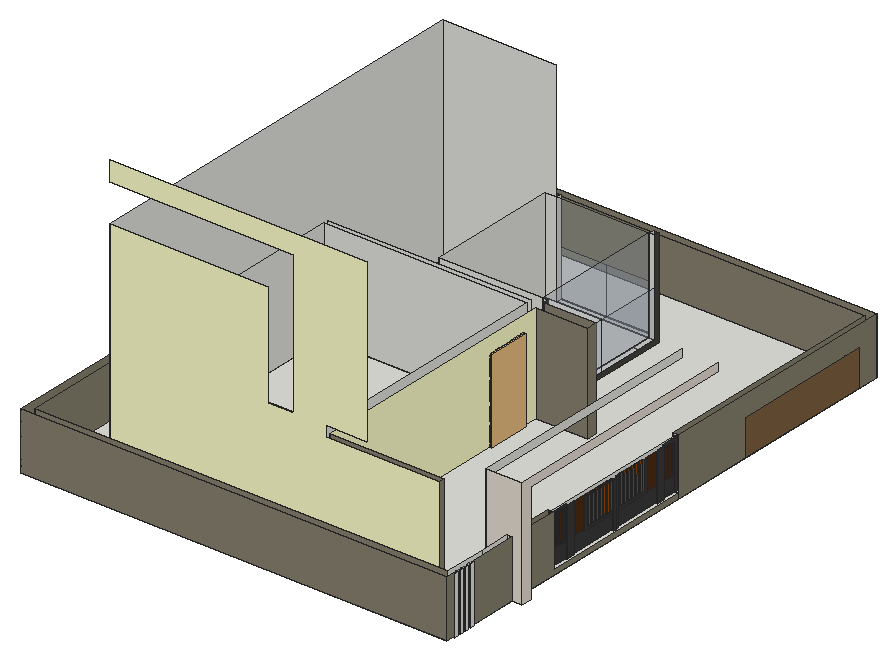
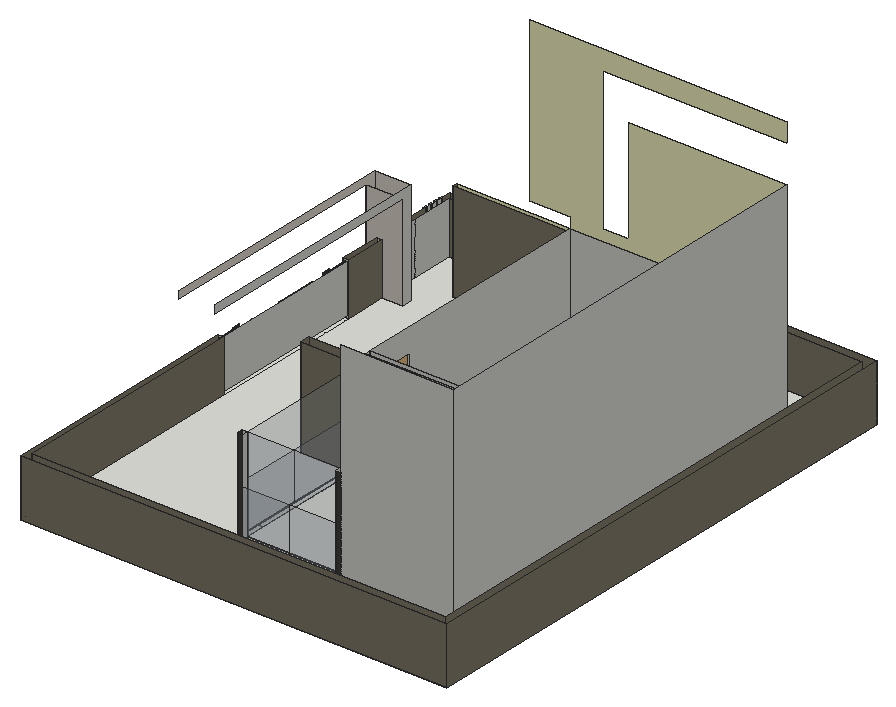
# SketchUp Ruby script. Lengths in inches.
U = 1.inch
M = Sketchup.active_model
def pt(a) = Geom::Point3d.new(a.map { |v| v * U })
def face(e, loops, mat)
  f = e.add_face(loops[0].map { |a| pt(a) })
  loops[1..].each { |l| e.add_face(l.map { |a| pt(a) }).erase! }
  f.material = f.back_material = mat if mat
  f
end
# faces: each face lists its corners as indices into pts; further lists are holes
def faces(e, pts, list, mat = nil) = list.each { |f| face(e, (f[0].is_a?(Array) ? f : [f]).map { |l| l.map { |i| pts[i] } }, mat) }
# xy, xz, yz: faces in a plane at the given z, y or x. An outline is a flat list of corners, or four numbers for a rectangle; further outlines are holes
def ring(l) = l.size == 4 ? [[l[0], l[1]], [l[2], l[1]], [l[2], l[3]], [l[0], l[3]]] : l.each_slice(2).to_a
def flat(e, list, mat, &to3) = list.each { |f| face(e, (f[0].is_a?(Array) ? f : [f]).map { |l| ring(l).map { |u, v| to3.(u, v) } }, mat) }
def xy(e, z, list, mat = nil) = flat(e, list, mat) { |x, y| [x, y, z] }
def xz(e, y, list, mat = nil) = flat(e, list, mat) { |x, z| [x, y, z] }
def yz(e, x, list, mat = nil) = flat(e, list, mat) { |y, z| [x, y, z] }
def lines(e, pts, list) = list.each { |a, b| e.add_line(pt(pts[a]), pt(pts[b])) }
# prism: a flat outline (further loops are holes) pulled along v
def prism(e, loops, v, mat = nil)
  f = face(e, loops, mat); d = Geom::Vector3d.new(v.map { |x| x * U })
  f.pushpull(f.normal.samedirection?(d) ? d.length : -d.length)
end
def box(e, o, s, mat = nil) = prism(e, [[o, [o[0] + s[0], o[1], o[2]], [o[0] + s[0], o[1] + s[1], o[2]], [o[0], o[1] + s[1], o[2]]]], [0, 0, s[2]], mat)
def at(x, y, z, deg = 0) = Geom::Transformation.translation(pt([x, y, z])) * Geom::Transformation.rotation(ORIGIN, Z_AXIS, deg.degrees)
def axes(o, x, y, z) = Geom::Transformation.new([*x, 0, *y, 0, *z, 0, *pt(o).to_a, 1])
def part(name) = M.definitions.add(name)
# library, detail: a bought-in or finely detailed component or shape, given as its bounding box
def library(name, o, s) = part(name).tap { |d| box(d.entities, o, s) }
def detail(e, o, s) = box(e.add_group.entities, o, s)
def put(e, d, t, mat = nil) = e.add_instance(d, t).tap { |i| i.material = mat if mat }
def group(e, t, mat = nil) = e.add_group.tap { |g| g.transformation = t; g.material = mat if mat }.entities
root = M.entities
M.materials.add("Brick_09_1K").color = [135, 129, 110]
M.materials.add("C07_Caramel_Shine").color = [153, 76, 0]
M.materials.add("E01_Mint_Frost").color = [255, 255, 204]
M.materials.add("Glass_Basic_01").color = [161, 173, 186]
M.materials["Glass_Basic_01"].alpha = 0.25
M.materials.add("Marble_01_1K").color = [230, 221, 211]
M.materials.add("Plywood_01_1K").color = [125, 96, 64]
M.materials.add("Wood_Planks_01_1K").color = [69, 67, 63]
M.materials.add("[Color_007]1").color = [58, 58, 58]
M.materials.add("[Wood_Cherry_Original]1").color = [76, 43, 21]
c1 = library("porta+4",[0.2,-5.42,1.33],[46.55,4.72,83.21])
xy(root,-6,[[0,0,0,618.14,492,618.14,492,35.25,494,35.25,494,31.5,492,31.5,492,27.75,494,27.75,494,24,492,24,492,20.25,494,20.25,494,16.5,492,16.5,492,12.75,494,12.75,494,9,492,9,492,0],[492,93,504,105]])
xy(root,0,[[[9,9,486,9,486,93,462,93,462,105,486,105,486,609.14,9,609.14],[57,57,57,537,306,537,306,372,366,372,366,360,306,360,306,63,438,63,438,57]],[[57,57,306,57,306,360,366,360,366,372,306,372,306,537,300,537,300,360,66,360,66,537,57,537],[66,66,300,354]],[66,66,300,354],[486,153,492,333],[66,360,300,537]])
xy(root,2,[[488,153,488,333,490,333,490,312.5,492,312.5,492,303.5,490,303.5,490,246,492,246,492,240,490,240,490,182.5,492,182.5,492,173.5,490,173.5,490,153]],"[Color_007]1")
xy(root,3,[[300,297,306,339]])
xy(root,6,[[180,378,300,531],[300,378,306,508.51],[300,508.51,306,531],[193.5,531,300,537]])
xy(root,9,[[210,360,252,378]])
xy(root,20,[[488,155,490,155.93],[488,156.85,490,157.78],[488,158.7,490,159.625],[488,160.55,490,161.48],[488,162.4,490,163.33],
  [488,164.25,490,165.18],[488,166.1,490,167.03],[488,167.95,490,168.875],[488,169.8,490,170.73],[488,171.65,490,172.58],
  [488,315.28,490,316.2],[488,317.125,490,318.05],[488,318.98,490,319.9],[488,320.83,490,321.75],[488,322.68,490,323.6],
  [488,324.53,490,325.45],[488,326.375,490,327.3],[488,328.23,490,329.15],[488,330.08,490,331]])
xy(root,20,[[490,198,492,240],[490,246,492,288]],"[Color_007]1")
xy(root,23,[[488,201.98,492,202.95],[488,203.92,492,204.9],[488,205.875,492,206.85],[488,207.83,492,208.8],[488,209.78,492,210.75],
  [488,211.73,492,212.7],[488,213.68,492,214.65],[488,215.625,492,216.6],[488,217.58,492,218.55],[488,219.53,492,220.5],
  [488,221.48,492,222.45],[488,223.42,492,224.4],[488,225.375,492,226.35],[488,227.33,492,228.3],[488,229.28,492,230.25],
  [488,231.23,492,232.2],[488,233.18,492,234.15],[488,235.125,492,236.1],[488,237.08,492,238.05],[488,239.03,492,240],
  [488,246,492,246.98],[488,247.95,492,248.92],[488,249.9,492,250.875],[488,251.85,492,252.83],[488,253.8,492,254.78],
  [488,255.75,492,256.73],[488,257.7,492,258.68],[488,259.65,492,260.625],[488,261.6,492,262.58],[488,263.55,492,264.53],
  [488,265.5,492,266.48],[488,267.45,492,268.42],[488,269.4,492,270.375],[488,271.35,492,272.33],[488,273.3,492,274.28],
  [488,275.25,492,276.23],[488,277.2,492,278.18],[488,279.15,492,280.125],[488,281.1,492,282.08],[488,283.05,492,284.03]])
xy(root,23,[[490,201,492,201.98],[490,202.95,492,203.92],[490,204.9,492,205.875],[490,206.85,492,207.83],[490,208.8,492,209.78],
  [490,210.75,492,211.73],[490,212.7,492,213.68],[490,214.65,492,215.625],[490,216.6,492,217.58],[490,218.55,492,219.53],
  [490,220.5,492,221.48],[490,222.45,492,223.42],[490,224.4,492,225.375],[490,226.35,492,227.33],[490,228.3,492,229.28],
  [490,230.25,492,231.23],[490,232.2,492,233.18],[490,234.15,492,235.125],[490,236.1,492,237.08],[490,238.05,492,239.03],
  [490,246.98,492,247.95],[490,248.92,492,249.9],[490,250.875,492,251.85],[490,252.83,492,253.8],[490,254.78,492,255.75],
  [490,256.73,492,257.7],[490,258.68,492,259.65],[490,260.625,492,261.6],[490,262.58,492,263.55],[490,264.53,492,265.5],
  [490,266.48,492,267.45],[490,268.42,492,269.4],[490,270.375,492,271.35],[490,272.33,492,273.3],[490,274.28,492,275.25],
  [490,276.23,492,277.2],[490,278.18,492,279.15],[490,280.125,492,281.1],[490,282.08,492,283.05],[490,284.03,492,285]],"[Color_007]1")
xz(root,0,[[0,-6,492,60]],"Brick_09_1K")
xz(root,9,[[492,-6,494,60]])
xz(root,9,[[9,0,486,60]],"Brick_09_1K")
xz(root,12.75,[[492,-6,494,60]])
xz(root,16.5,[[492,-6,494,60]])
xz(root,20.25,[[492,-6,494,60]])
xz(root,24,[[492,-6,494,60]])
xz(root,27.75,[[492,-6,494,60]])
xz(root,31.5,[[492,-6,494,60]])
xz(root,35.25,[[492,-6,494,60]])
xz(root,57,[[57,0,438,0,438,114,306,114,306,126,354,126,354,312,57,312,57,289.5,270,289.5,270,126,240,126,240,246,57,246]],"E01_Mint_Frost")
xz(root,63,[[306,0,438,114]],"Brick_09_1K")
xz(root,66,[[66,0,300,120]])
xz(root,93,[[492,-6,504,-6,504,120,462,120,462,0,486,0,486,60,492,60]],"Marble_01_1K")
xz(root,105,[[492,-6,492,60,486,60,486,0,462,0,462,111,504,111,504,-6]],"Marble_01_1K")
xz(root,153,[[[486,0,492,60],[488,2,490,58]]])
xz(root,155,[[488,20,490,22],[488,22,490,55.99]])
xz(root,155.93,[[488,20,490,22],[488,22,490,55.98]])
xz(root,156.85,[[488,20,490,22],[488,22,490,55.98]])
xz(root,157.78,[[488,20,490,22],[488,22,490,55.97]])
xz(root,158.7,[[488,20,490,22],[488,22,490,55.97]])
xz(root,159.625,[[488,20,490,22],[488,22,490,55.96]])
xz(root,160.55,[[488,20,490,22],[488,22,490,55.96]])
xz(root,161.48,[[488,20,490,22],[488,22,490,55.95]])
xz(root,162.4,[[488,20,490,22],[488,22,490,55.95]])
xz(root,163.33,[[488,20,490,22.01],[488,22.01,490,55.94]])
xz(root,164.25,[[488,20,490,22.01],[488,22.01,490,55.9375]])
xz(root,165.18,[[488,20,490,22.01],[488,22.01,490,55.93]])
xz(root,166.1,[[488,20,490,22.01],[488,22.01,490,55.93]])
xz(root,167.03,[[488,20,490,22.01],[488,22.01,490,55.92]])
xz(root,167.95,[[488,20,490,22.01],[488,22.01,490,55.92]])
xz(root,168.875,[[488,20,490,22.01],[488,22.01,490,55.91]])
xz(root,169.8,[[488,20,490,22.01],[488,22.01,490,55.91]])
xz(root,170.73,[[488,20,490,22.01],[488,22.01,490,55.9]])
xz(root,171.65,[[488,20,490,22.01],[488,22.01,490,55.9]])
xz(root,172.58,[[488,20,490,22.01],[488,22.01,490,55.89]])
xz(root,173.5,[[490,2,492,20],[490,20,492,22],[490,22,492,58]],"[Color_007]1")
xz(root,182.5,[[490,2,492,55.84]],"[Color_007]1")
xz(root,198,[[490,20,492,55.75]],"[Color_007]1")
xz(root,201,[[490,23,492,55]],"[Color_007]1")
xz(root,201.98,[[488,23,490,55]],"[Color_007]1")
xz(root,202.95,[[488,23,490,55]],"[Color_007]1")
xz(root,203.92,[[488,23,490,55]],"[Color_007]1")
xz(root,204.9,[[488,23,490,55]],"[Color_007]1")
xz(root,205.875,[[488,23,490,55]],"[Color_007]1")
xz(root,206.85,[[488,23,490,55]],"[Color_007]1")
xz(root,207.83,[[488,23,490,55]],"[Color_007]1")
xz(root,208.8,[[488,23,490,55]],"[Color_007]1")
xz(root,209.78,[[488,23,490,55]],"[Color_007]1")
xz(root,210.75,[[488,23,490,55]],"[Color_007]1")
xz(root,211.73,[[488,23,490,55]],"[Color_007]1")
xz(root,212.7,[[488,23,490,55]],"[Color_007]1")
xz(root,213.68,[[488,23,490,55]],"[Color_007]1")
xz(root,214.65,[[488,23,490,55]],"[Color_007]1")
xz(root,215.625,[[488,23,490,55]],"[Color_007]1")
xz(root,216.6,[[488,23,490,55]],"[Color_007]1")
xz(root,217.58,[[488,23,490,55]],"[Color_007]1")
xz(root,218.55,[[488,23,490,55]],"[Color_007]1")
xz(root,219.53,[[488,23,490,55]],"[Color_007]1")
xz(root,220.5,[[488,23,490,55]],"[Color_007]1")
xz(root,221.48,[[488,23,490,55]],"[Color_007]1")
xz(root,222.45,[[488,23,490,55]],"[Color_007]1")
xz(root,223.42,[[488,23,490,55]],"[Color_007]1")
xz(root,224.4,[[488,23,490,55]],"[Color_007]1")
xz(root,225.375,[[488,23,490,55]],"[Color_007]1")
xz(root,226.35,[[488,23,490,55]],"[Color_007]1")
xz(root,227.33,[[488,23,490,55]],"[Color_007]1")
xz(root,228.3,[[488,23,490,55]],"[Color_007]1")
xz(root,229.28,[[488,23,490,55]],"[Color_007]1")
xz(root,230.25,[[488,23,490,55]],"[Color_007]1")
xz(root,231.23,[[488,23,490,55]],"[Color_007]1")
xz(root,232.2,[[488,23,490,55]],"[Color_007]1")
xz(root,233.18,[[488,23,490,55]],"[Color_007]1")
xz(root,234.15,[[488,23,490,55]],"[Color_007]1")
xz(root,235.125,[[488,23,490,55]],"[Color_007]1")
xz(root,236.1,[[488,23,490,55]],"[Color_007]1")
xz(root,237.08,[[488,23,490,55]],"[Color_007]1")
xz(root,238.05,[[488,23,490,55]],"[Color_007]1")
xz(root,239.03,[[488,23,490,55]])
xz(root,240,[[490,2,492,20],[488,23,492,55]],"[Color_007]1")
xz(root,246,[[490,2,492,20],[488,23,492,55]],"[Color_007]1")
xz(root,246.98,[[488,23,490,55]])
xz(root,247.95,[[488,23,490,55]],"[Color_007]1")
xz(root,248.92,[[488,23,490,55]],"[Color_007]1")
xz(root,249.9,[[488,23,490,55]],"[Color_007]1")
xz(root,250.875,[[488,23,490,55]],"[Color_007]1")
xz(root,251.85,[[488,23,490,55]],"[Color_007]1")
xz(root,252.83,[[488,23,490,55]],"[Color_007]1")
xz(root,253.8,[[488,23,490,55]],"[Color_007]1")
xz(root,254.78,[[488,23,490,55]],"[Color_007]1")
xz(root,255.75,[[488,23,490,55]],"[Color_007]1")
xz(root,256.73,[[488,23,490,55]],"[Color_007]1")
xz(root,257.7,[[488,23,490,55]],"[Color_007]1")
xz(root,258.68,[[488,23,490,55]],"[Color_007]1")
xz(root,259.65,[[488,23,490,55]],"[Color_007]1")
xz(root,260.625,[[488,23,490,55]],"[Color_007]1")
xz(root,261.6,[[488,23,490,55]],"[Color_007]1")
xz(root,262.58,[[488,23,490,55]],"[Color_007]1")
xz(root,263.55,[[488,23,490,55]],"[Color_007]1")
xz(root,264.53,[[488,23,490,55]],"[Color_007]1")
xz(root,265.5,[[488,23,490,55]],"[Color_007]1")
xz(root,266.48,[[488,23,490,55]],"[Color_007]1")
xz(root,267.45,[[488,23,490,55]],"[Color_007]1")
xz(root,268.42,[[488,23,490,55]],"[Color_007]1")
xz(root,269.4,[[488,23,490,55]],"[Color_007]1")
xz(root,270.375,[[488,23,490,55]],"[Color_007]1")
xz(root,271.35,[[488,23,490,55]],"[Color_007]1")
xz(root,272.33,[[488,23,490,55]],"[Color_007]1")
xz(root,273.3,[[488,23,490,55]],"[Color_007]1")
xz(root,274.28,[[488,23,490,55]],"[Color_007]1")
xz(root,275.25,[[488,23,490,55]],"[Color_007]1")
xz(root,276.23,[[488,23,490,55]],"[Color_007]1")
xz(root,277.2,[[488,23,490,55]],"[Color_007]1")
xz(root,278.18,[[488,23,490,55]],"[Color_007]1")
xz(root,279.15,[[488,23,490,55]],"[Color_007]1")
xz(root,280.125,[[488,23,490,55]],"[Color_007]1")
xz(root,281.1,[[488,23,490,55]],"[Color_007]1")
xz(root,282.08,[[488,23,490,55]],"[Color_007]1")
xz(root,283.05,[[488,23,490,55]],"[Color_007]1")
xz(root,284.03,[[488,23,490,55]],"[Color_007]1")
xz(root,285,[[490,23,492,55]],"[Color_007]1")
xz(root,288,[[490,20,492,55]],"[Color_007]1")
xz(root,297,[[300,3,306,93]])
xz(root,303.5,[[490,2,492,4],[490,4,492,20],[490,20,492,55.16]],"[Color_007]1")
xz(root,312.5,[[490,2,492,58]],"[Color_007]1")
xz(root,313.42,[[488,20.01,490,20.1]])
xz(root,313.42,[[488,20.1,490,55]],"[Color_007]1")
xz(root,314.35,[[488,20,490,20.1]])
xz(root,314.35,[[488,20.1,490,55]],"[Color_007]1")
xz(root,315.28,[[488,20,490,20.1]])
xz(root,315.28,[[488,20.1,490,55]],"[Color_007]1")
xz(root,316.2,[[488,20,490,20.1]])
xz(root,316.2,[[488,20.1,490,54.98]],"[Color_007]1")
xz(root,317.125,[[488,20,490,20.1]])
xz(root,317.125,[[488,20.1,490,54.98]],"[Color_007]1")
xz(root,318.05,[[488,20,490,20.1]])
xz(root,318.05,[[488,20.1,490,54.98]],"[Color_007]1")
xz(root,318.98,[[488,20,490,20.1]])
xz(root,318.98,[[488,20.1,490,54.98]],"[Color_007]1")
xz(root,319.9,[[488,20,490,20.1]])
xz(root,319.9,[[488,20.1,490,54.98]],"[Color_007]1")
xz(root,320.83,[[488,20,490,20.1]])
xz(root,320.83,[[488,20.1,490,54.98]],"[Color_007]1")
xz(root,321.75,[[488,20,490,20.1]])
xz(root,321.75,[[488,20.1,490,54.98]],"[Color_007]1")
xz(root,322.68,[[488,20,490,20.1]])
xz(root,322.68,[[488,20.1,490,54.98]],"[Color_007]1")
xz(root,323.6,[[488,20,490,20.1]])
xz(root,323.6,[[488,20.1,490,54.98]],"[Color_007]1")
xz(root,324.53,[[488,20,490,20.1]])
xz(root,324.53,[[488,20.1,490,54.98]],"[Color_007]1")
xz(root,325.45,[[488,20,490,20.1]])
xz(root,325.45,[[488,20.1,490,54.98]],"[Color_007]1")
xz(root,326.375,[[488,20,490,20.1]])
xz(root,326.375,[[488,20.1,490,54.98]],"[Color_007]1")
xz(root,327.3,[[488,20,490,20.1]])
xz(root,327.3,[[488,20.1,490,54.98]],"[Color_007]1")
xz(root,328.23,[[488,20,490,20.1]])
xz(root,328.23,[[488,20.1,490,54.98]],"[Color_007]1")
xz(root,329.15,[[488,20,490,20.1]])
xz(root,329.15,[[488,20.1,490,54.98]],"[Color_007]1")
xz(root,330.08,[[488,20,490,20.1]])
xz(root,330.08,[[488,20.1,490,54.98]],"[Color_007]1")
xz(root,331,[[488,20,490,20.1]])
xz(root,331,[[488,20.1,490,54.98]],"[Color_007]1")
xz(root,333,[[[486,0,492,60],[488,2,490,58]]])
xz(root,339,[[300,3,306,93]])
xz(root,354,[[66,0,300,120]])
xz(root,360,[[[66,0,300,120],[210,9,252,87]]])
xz(root,360,[[306,0,366,114]],"Brick_09_1K")
xz(root,372,[[306,0,366,114]],"Brick_09_1K")
xz(root,378,[[180,6,180,114,300,114,300,6,255,6,255,90,207,90,207,6],[[207,6,255,90],[210,9,252,87]],[300,6,306,114]])
xz(root,531,[[180,6,193.5,114],[300,6,306,114]])
xz(root,531,[[193.5,6,300,114]],"Glass_Basic_01")
xz(root,537,[[57,0,187.5,246]])
xz(root,537,[[193.5,6,246.75,60],[246.75,6,300,60]],"Glass_Basic_01")
xz(root,537,[[187.5,0,187.5,114,193.5,114,193.5,6,300,6,300,114,306,114,306,0]],"Wood_Planks_01_1K")
xz(root,609.14,[[9,0,486,60]],"Brick_09_1K")
xz(root,618.14,[[0,-6,492,60]],"Brick_09_1K")
yz(root,0,[[0,-6,618.14,60]],"Brick_09_1K")
yz(root,9,[[9,0,609.14,60]],"Brick_09_1K")
yz(root,57,[[57,0,537,246]])
yz(root,66,[[66,0,354,120]])
yz(root,180,[[378,6,531,114]])
yz(root,193.5,[[531,6,537,114]])
yz(root,210,[[360,9,378,87]])
yz(root,252,[[360,9,378,87]])
yz(root,300,[[[66,0,354,120],[297,3,339,93]],[531,6,537,114]])
yz(root,300,[[378,6,531,114]],"Glass_Basic_01")
yz(root,306,[[[294,0,342,96],[297,3,339,93]]])
yz(root,306,[[63,0,294,0,294,96,342,96,342,0,360,0,360,114,63,114]],"E01_Mint_Frost")
yz(root,306,[[378,6,454.5,60],[454.5,6,531,60]],"Glass_Basic_01")
yz(root,306,[[372,0,537,0,537,114,531,114,531,6,378,6,378,114,372,114]],"Wood_Planks_01_1K")
yz(root,366,[[360,0,372,114]],"Brick_09_1K")
yz(root,438,[[57,0,63,114]],"Brick_09_1K")
yz(root,462,[[93,0,93,120,375,120,375,111,105,111,105,0]])
yz(root,486,[[9,0,57,60],[57,0,93,60]])
yz(root,486,[[105,0,153,60],[333,0,609.14,60]],"Brick_09_1K")
yz(root,488,[[[153,2,333,58],[155,20,155.93,20,155.93,55.98,155,55.99],[156.85,20,157.78,20,157.78,55.97,156.85,55.98],[158.7,20,159.625,20,159.625,55.96,158.7,55.97],[160.55,20,161.48,20,161.48,55.95,160.55,55.96],[162.4,20,163.33,20,163.33,55.94,162.4,55.95],[164.25,20,165.18,20,165.18,55.93,164.25,55.9375],[166.1,20,167.03,20,167.03,55.92,166.1,55.93],[167.95,20,168.875,20,168.875,55.91,167.95,55.92],[169.8,20,170.73,20,170.73,55.9,169.8,55.91],[171.65,20,172.58,20,172.58,55.89,171.65,55.9],[314.35,20,314.35,55.1,313.42,55.11,313.42,20.01],[315.28,20,316.2,20,316.2,55.09,315.28,55.1],[317.125,20,318.05,20,318.05,55.08,317.125,55.09],[318.98,20,319.9,20,319.9,55.07,318.98,55.08],[320.83,20,321.75,20,321.75,55.0625,320.83,55.07],[322.68,20,323.6,20,323.6,55.05,322.68,55.06],[324.53,20,325.45,54.98],[326.375,20,327.3,54.98],[328.23,20,329.15,54.98],[330.08,20,331,54.98],[201.98,23,202.95,55],[203.92,23,204.9,55],[205.875,23,206.85,55],[209.78,23,210.75,55],[211.73,23,212.7,55],[213.68,23,214.65,55],[215.625,23,216.6,55],[219.53,23,220.5,55],[221.48,23,222.45,55],[223.42,23,224.4,55],[225.375,23,226.35,55],[229.28,23,230.25,55],[231.23,23,232.2,55],[235.125,23,236.1,55],[239.03,23,240,55],[237.08,23,238.05,55],[246,23,246.98,55],[249.9,23,250.875,55],[251.85,23,252.83,55],[253.8,23,254.78,55],[255.75,23,256.73,55],[259.65,23,260.625,55],[261.6,23,262.58,55],[263.55,23,264.53,55],[265.5,23,266.48,55],[269.4,23,270.375,55],[271.35,23,272.33,55],[273.3,23,274.28,55],[275.25,23,276.23,55],[277.2,23,278.18,55],[279.15,23,280.125,55],[281.1,23,282.08,55],[207.83,23,208.8,55],[217.58,23,218.55,55],[227.33,23,228.3,55],[233.18,23,234.15,55],[247.95,23,248.92,55],[257.7,23,258.68,55],[267.45,23,268.42,55],[283.05,23,284.03,55]]])
yz(root,490,[[313.42,20,314.35,20,313.42,20.01],[313.21,20.01,313.42,20.01,313.42,55]])
yz(root,490,[[201,23,201.98,55],[202.95,23,203.92,55],[204.9,23,205.875,55],[206.85,23,207.83,55],[208.8,23,209.78,55],
  [210.75,23,211.73,55],[212.7,23,213.68,55],[214.65,23,215.625,55],[216.6,23,217.58,55],[218.55,23,219.53,55],
  [220.5,23,221.48,55],[222.45,23,223.42,55],[224.4,23,225.375,55],[226.35,23,227.33,55],[228.3,23,229.28,55],
  [230.25,23,231.23,55],[232.2,23,233.18,55],[234.15,23,235.125,55],[236.1,23,237.08,55],[238.05,23,239.03,55],
  [246.98,23,247.95,55],[248.92,23,249.9,55],[250.875,23,251.85,55],[252.83,23,253.8,55],[254.78,23,255.75,55],
  [256.73,23,257.7,55],[258.68,23,259.65,55],[260.625,23,261.6,55],[262.58,23,263.55,55],[264.53,23,265.5,55],
  [266.48,23,267.45,55],[268.42,23,269.4,55],[270.375,23,271.35,55],[272.33,23,273.3,55],[274.28,23,275.25,55],
  [276.23,23,277.2,55],[278.18,23,279.15,55],[280.125,23,281.1,55],[282.08,23,283.05,55],[284.03,23,285,55]],"C07_Caramel_Shine")
yz(root,490,[[153,2,173.5,20],[182.5,2,240,20],[246,2,303.5,20],[312.5,2,333,2,333,20,331,20,331,4,312.5,4],[312.5,4,331,20],
  [153,20,155,20,155,56,173.5,56,173.5,58,153,58],[331,20,333,20,333,58,312.5,58,312.5,55.11,313.42,55.11,314.35,55.1,315.28,55.1,316.2,55.09,317.125,55.09,318.05,55.08,318.98,55.08,319.9,55.07,320.83,55.07,321.75,55.0625,322.68,55.06,323.6,55.05,324.53,55.05,325.45,55.04,326.375,55.04,327.3,55.03,328.23,55.03,329.15,55.02,330.08,55.02,331,55.01]],"[Color_007]1")
yz(root,490,[[155.93,20,156.85,55.98],[157.78,20,158.7,55.97],[159.625,20,160.55,55.96],[161.48,20,162.4,55.95],[163.33,20,164.25,20,164.25,55.9375,163.33,55.94],
  [165.18,20,166.1,55.93],[167.03,20,167.95,55.92],[168.875,20,169.8,55.91],[170.73,20,171.65,55.9],[172.58,20,173.5,55.89],
  [182.5,20,198,20,198,55.75,182.5,55.84],[288,20,303.5,55],[312.5,20,313.42,20,313.42,20.01,313.21,20.01,313.42,55,313.42,55.11,312.5,55.11],[314.35,20,315.28,20,315.28,55.1,314.5625,55.1,314.35,20.1],[316.2,20,317.125,55.09],
  [318.05,20,318.98,55.08],[319.9,20,320.83,55.07],[321.75,20,322.68,20,322.68,55.06,321.75,55.0625],[323.6,20,324.53,55.05],[325.45,20,326.375,54.98],
  [327.3,20,328.23,54.98],[329.15,20,330.08,54.98],[314.35,20.1,314.5625,55.1,314.35,55.1]],"[Wood_Cherry_Original]1")
yz(root,492,[[12.75,-6,16.5,60],[20.25,-6,24,60],[27.75,-6,31.5,60]])
yz(root,492,[[0,-6,9,60],[35.25,-6,93,60],[105,-6,333,-6,333,0,153,0,153,60,105,60],[333,-6,429,-6,429,36,594.14,36,594.14,-6,618.14,-6,618.14,60,333,60]],"Brick_09_1K")
yz(root,492,[[429,-6,594.14,36]],"Plywood_01_1K")
yz(root,492,[[173.5,2,182.5,58],[240,2,243,2,243,55.5,240,55.52],[243,2,246,2,246,55.48,243,55.5],[303.5,2,312.5,58],[198,20,240,20,240,23,201,23,201,55,240,55,240,55.52,198,55.75],
  [246,20,288,20,288,55,285,55,285,23,246,23]],"[Color_007]1")
yz(root,494,[[9,-6,12.75,60],[16.5,-6,20.25,60],[24,-6,27.75,60],[31.5,-6,35.25,60]])
yz(root,504,[[93,-6,105,-6,105,111,375,111,375,120,93,120]],"Marble_01_1K")
p = [[490,313.42,20.01],[490,314.35,20],[488,314.35,20],[488,313.42,20.01],[306,66,0],[300,66,0],
  [486,609.14,0],[486,618.14,0]]
faces(root,p,[[0,1,2,3]])
lines(root,p,[[4,5],[6,7]])
put(root,c1,axes([303.24,293.79,-1.54],[0,1.03118,0],[-1,0,0],[0,0,1.15408]))
put(root,c1,axes([255.21,376.16,4.45],[-1.03118,0,0],[0,-1,0],[0,0,1.15408]))
